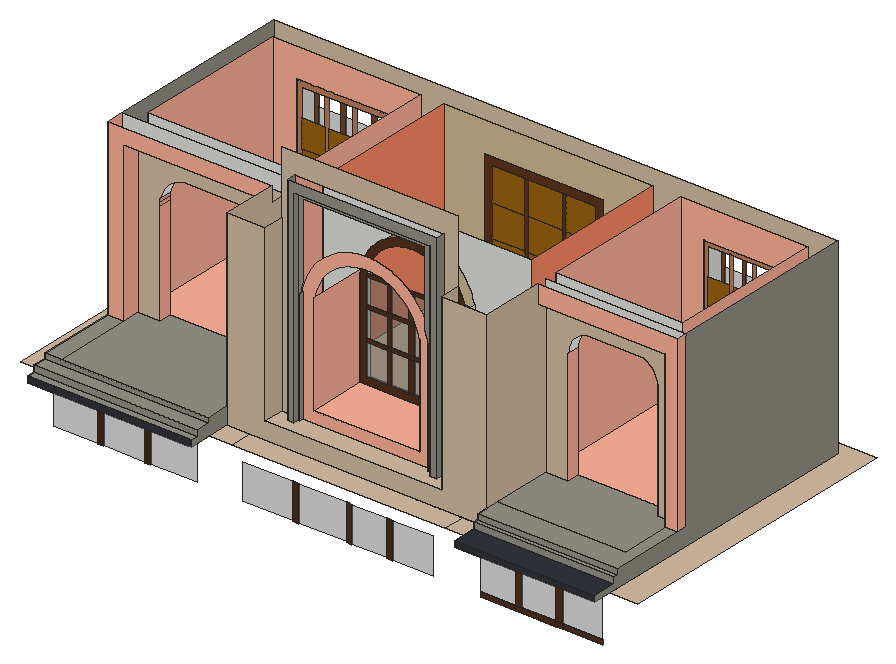
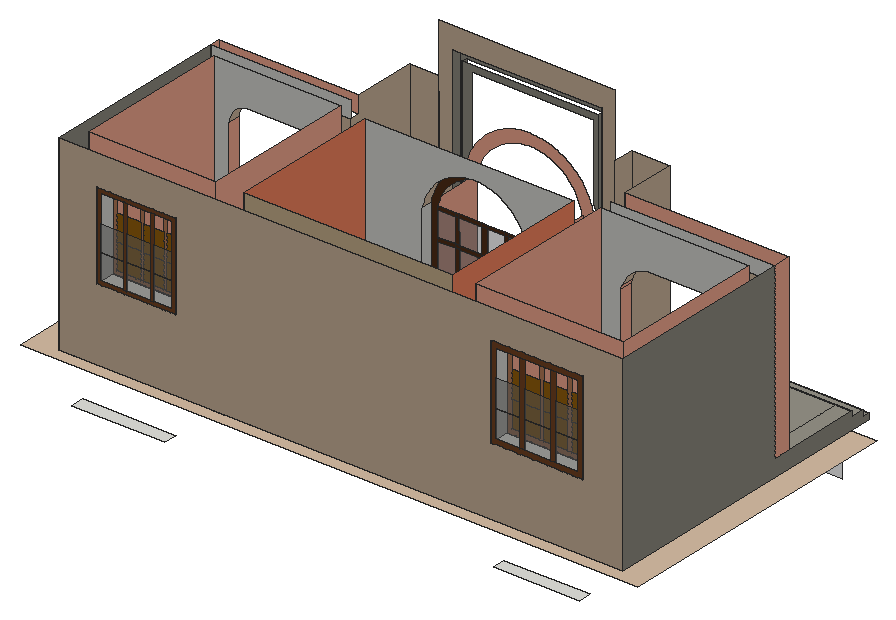
# SketchUp Ruby script. Lengths in inches.
U = 1.inch
M = Sketchup.active_model
def pt(a) = Geom::Point3d.new(a.map { |v| v * U })
def face(e, loops, mat)
  f = e.add_face(loops[0].map { |a| pt(a) })
  loops[1..].each { |l| e.add_face(l.map { |a| pt(a) }).erase! }
  f.material = f.back_material = mat if mat
  f
end
# faces: each face lists its corners as indices into pts; further lists are holes
def faces(e, pts, list, mat = nil) = list.each { |f| face(e, (f[0].is_a?(Array) ? f : [f]).map { |l| l.map { |i| pts[i] } }, mat) }
# xy, xz, yz: faces in a plane at the given z, y or x. An outline is a flat list of corners, or four numbers for a rectangle; further outlines are holes
def ring(l) = l.size == 4 ? [[l[0], l[1]], [l[2], l[1]], [l[2], l[3]], [l[0], l[3]]] : l.each_slice(2).to_a
def flat(e, list, mat, &to3) = list.each { |f| face(e, (f[0].is_a?(Array) ? f : [f]).map { |l| ring(l).map { |u, v| to3.(u, v) } }, mat) }
def xy(e, z, list, mat = nil) = flat(e, list, mat) { |x, y| [x, y, z] }
def xz(e, y, list, mat = nil) = flat(e, list, mat) { |x, z| [x, y, z] }
def yz(e, x, list, mat = nil) = flat(e, list, mat) { |y, z| [x, y, z] }
def lines(e, pts, list) = list.each { |a, b| e.add_line(pt(pts[a]), pt(pts[b])) }
# prism: a flat outline (further loops are holes) pulled along v
def prism(e, loops, v, mat = nil)
  f = face(e, loops, mat); d = Geom::Vector3d.new(v.map { |x| x * U })
  f.pushpull(f.normal.samedirection?(d) ? d.length : -d.length)
end
def box(e, o, s, mat = nil) = prism(e, [[o, [o[0] + s[0], o[1], o[2]], [o[0] + s[0], o[1] + s[1], o[2]], [o[0], o[1] + s[1], o[2]]]], [0, 0, s[2]], mat)
def at(x, y, z, deg = 0) = Geom::Transformation.translation(pt([x, y, z])) * Geom::Transformation.rotation(ORIGIN, Z_AXIS, deg.degrees)
def axes(o, x, y, z) = Geom::Transformation.new([*x, 0, *y, 0, *z, 0, *pt(o).to_a, 1])
def part(name) = M.definitions.add(name)
# library, detail: a bought-in or finely detailed component or shape, given as its bounding box
def library(name, o, s) = part(name).tap { |d| box(d.entities, o, s) }
def detail(e, o, s) = box(e.add_group.entities, o, s)
def put(e, d, t, mat = nil) = e.add_instance(d, t).tap { |i| i.material = mat if mat }
def group(e, t, mat = nil) = e.add_group.tap { |g| g.transformation = t; g.material = mat if mat }.entities
root = M.entities
M.materials.add("[Blinds Wood Light]").color = [155, 100, 14]
M.materials.add("[Color B02]").color = [255, 178, 153]
M.materials.add("[Color B03]").color = [255, 140, 101]
M.materials.add("[Formica Beige]").color = [211, 187, 149]
M.materials.add("[Formica Graystone]").color = [149, 146, 135]
M.materials.add("[Formica Laminate Dark]").color = [50, 53, 60]
M.materials.add("[Formica Laminate Light]").color = [213, 189, 164]
M.materials.add("[Translucent Glass Gray]").color = [128, 128, 128]
M.materials["[Translucent Glass Gray]"].alpha = 0.5
M.materials.add("[Wood Cherry Original]").color = [152, 86, 42]
M.materials.add("[Wood Veneer 01]").color = [71, 41, 22]
M.materials.add("[Wood Veneer 01]1").color = [84, 49, 25]
M.materials.add("[Wood Veneer 01]2").color = [94, 55, 29]
M.materials.add("[Wood Veneer 01]3").color = [84, 49, 25]
M.materials.add("[Wood Veneer 01]4").color = [79, 46, 24]
M.materials.add("[Wood Veneer 01]5").color = [120, 70, 37]
M.materials.add("[Wood Veneer 02]").color = [190, 128, 91]
xy(root,103.85,[[328.4,583.14,393.03,592.14]])
xy(root,106.46,[[40.61,583.14,100.11,592.14]])
xy(root,129,[[128.66,369.56,131.42,385.12],[128.66,385.12,128.66,583.14,146.72,583.14,146.72,400.56,131.42,400.56,131.42,385.12],[311.91,385.12,311.91,400.56,294.66,400.56,294.66,583.14,314.84,583.14,314.84,385.12],[146.72,474.18,294.66,484.13],[146.72,474.18,294.66,484.13]])
xy(root,129,[[17.625,385.12,128.66,583.14],[314.84,385.12,409.38,583.14]],"[Color B02]")
xy(root,129,[[17.625,369.56,128.66,385.12],[311.91,372.18,314.84,385.12],[314.84,372.18,409.38,385.12]],"[Formica Laminate Dark]")
xy(root,129,[[0,385.12,17.625,385.12,17.625,583.14,409.38,583.14,409.38,385.12,428.94,385.12,428.94,592.14,0,592.14],[131.42,385.12,146.72,400.56],[146.72,385.12,294.66,400.56],[294.66,385.12,311.91,400.56]],"[Formica Laminate Light]")
xy(root,129,[[146.72,400.56,294.66,474.18],[146.72,484.13,294.66,583.14]],"[Wood Cherry Original]")
xy(root,133.17,[[311.91,372.18,409.38,388.75]],"[Formica Laminate Dark]")
xy(root,133.35,[[17.625,369.56,131.42,374.93]],"[Formica Graystone]")
xy(root,137.33,[[311.91,388.75,409.38,392.06]],"[Formica Graystone]")
xy(root,137.7,[[17.625,374.93,131.42,384.31]],"[Formica Graystone]")
xy(root,141,[[17.625,438.8,28.78,451.42],[400.54,444.11,409.38,451.42]])
xy(root,141,[[28.78,459.89,131.42,568.57],[311.91,459.89,400.54,568.57]],"[Color B02]")
xy(root,141,[[147.71,463.02,292.81,568.57]],"[Formica Beige]")
xy(root,141,[[17.625,384.31,28.78,438.8],[28.78,384.31,131.42,384.31,131.42,451.42,117.53,451.42,117.53,459.89,43.6875,459.89,43.6875,451.42,28.78,451.42],[311.91,392.06,409.38,392.06,409.38,444.11,400.54,444.11,400.54,409.77,311.91,409.77],[311.91,409.77,400.54,409.77,400.54,451.42,389.71,451.42,389.71,459.89,327.58,459.89,327.58,451.42,311.91,451.42]],"[Formica Graystone]")
xy(root,141,[[157.59,400.56,280.13,400.56,280.13,414.84,270.12,414.84,270.12,408.78,265.76,408.78,265.76,412.53,261.39,412.53,261.39,414.84,172.21,414.84,172.21,412.53,170.76,412.53,170.76,408.78,166.89,408.78,166.89,414.84,157.59,414.84]],"[Formica Laminate Light]")
xy(root,149.01,[[180.21,454.92,253.39,463.02]])
xy(root,149.01,[[180.21,414.84,253.39,454.92]],"[Color B02]")
xy(root,176.09,[[45.27,568.57,109.65,583.14]])
xy(root,178.98,[[327.9375,568.57,383.25,583.14]])
xz(root,369.56,[[17.625,129,131.42,133.35]],"[Formica Laminate Dark]")
xz(root,372.18,[[311.91,129,409.38,133.17]],"[Formica Laminate Dark]")
xz(root,374.93,[[17.625,133.35,131.42,137.7]],"[Formica Graystone]")
xz(root,384.31,[[17.625,137.7,131.42,141]],"[Formica Graystone]")
xz(root,385.12,[[154.41,96.38,189.27,121.31],[193.22,96.38,226.58,121.31],[230.53,96.38,254.8,121.31],[258.75,96.38,286.96,121.31],[22.98,96.89,53.7,123.64],
  [57.87,96.89,86.41,123.64],[90.59,96.89,123.3,123.64],[319.73,98.41,344.24,124.11],[348.55,98.41,372.21,124.11],[376.51,98.41,404.48,124.11]],"[Translucent Glass Gray]")
xz(root,385.12,[[53.7,96.89,57.87,123.64],[86.41,96.89,90.59,123.64]],"[Wood Veneer 01]")
xz(root,385.12,[[319.73,95.2,344.24,98.41],[344.24,95.2,348.55,98.41],[348.55,95.2,372.21,98.41],[372.21,95.2,376.51,98.41],[376.51,95.2,404.48,98.41],
  [344.24,98.41,348.55,124.11],[372.21,98.41,376.51,124.11]],"[Wood Veneer 01]1")
xz(root,385.12,[[189.27,96.38,193.22,121.31],[226.58,96.38,230.53,121.31],[254.8,96.38,258.75,121.31]],"[Wood Veneer 01]4")
xz(root,388.75,[[311.91,133.17,409.38,137.33]],"[Formica Graystone]")
xz(root,392.06,[[311.91,137.33,409.38,141]],"[Formica Graystone]")
xz(root,400.56,[[131.42,129,311.91,129,311.91,261,280.13,261,280.13,141,157.59,141,157.59,261,131.42,261]],"[Formica Laminate Light]")
xz(root,408.78,[[166.89,141,170.76,141,170.76,284,265.76,284,265.76,141,270.12,141,270.12,290.79,166.89,290.79]],"[Formica Graystone]")
xz(root,412.53,[[170.76,141,172.21,141,172.21,219.8125,172.61,221.89,173.11,223.94,173.71,225.97,174.14,227.22,174.14,279.69,259.2,279.69,259.2,227.97,259.89,225.97,260.49,223.94,260.99,221.89,261.39,219.8125,261.39,141,265.76,141,265.76,284,170.76,284]],"[Formica Graystone]")
xz(root,414.84,[[[172.21,141,261.39,141,261.39,219.8125,260.99,221.89,260.49,223.94,259.89,225.97,259.2,227.97,258.42,229.93,257.55,231.85,256.58,233.73,255.53,235.57,254.4,237.35,253.18,239.08,251.89,240.75,250.52,242.36,249.07,243.9,247.56,245.375,245.97,246.77,244.33,248.1,242.62,249.34,240.86,250.51,239.04,251.59,237.18,252.59,235.27,253.49,233.32,254.3125,231.33,255.04,229.32,255.67,227.27,256.21,225.21,256.65,223.12,256.99,221.02,257.24,218.91,257.39,216.8,257.44,214.6875,257.39,212.58,257.24,210.48,256.99,208.39,256.65,206.33,256.21,204.28,255.67,202.27,255.04,200.28,254.3125,198.33,253.49,196.42,252.59,194.56,251.59,192.74,250.51,190.98,249.34,189.27,248.1,187.63,246.77,186.04,245.375,184.53,243.9,183.08,242.36,181.71,240.75,180.42,239.08,179.2,237.35,178.07,235.57,177.02,233.73,176.05,231.85,175.18,229.93,174.4,227.97,174.14,227.22,173.71,225.97,173.11,223.94,172.61,221.89,172.21,219.8125],[180.21,149.01,180.21,219.04,180.43,220.17,180.84,221.86,181.34,223.53,181.9,225.17,182.55,226.79,183.27,228.375,184.06,229.92,184.92,231.43,185.86,232.9,186.86,234.32,187.92,235.7,189.05,237.02,190.24,238.29,191.49,239.5,192.79,240.65,194.15,241.74,195.55,242.77,197,243.73,198.5,244.62,200.03,245.4375,201.6,246.18,203.21,246.86,204.84,247.45,206.5,247.97,208.18,248.42,209.88,248.78,211.6,249.0625,213.33,249.27,215.0625,249.39,216.8,249.43,218.54,249.39,220.27,249.27,222,249.0625,223.72,248.78,225.42,248.42,227.1,247.97,228.76,247.45,230.39,246.86,232,246.18,233.57,245.4375,235.1,244.62,236.6,243.73,238.05,242.77,239.45,241.74,240.81,240.65,242.11,239.5,243.36,238.29,244.55,237.02,245.68,235.7,246.74,234.32,247.74,232.9,248.68,231.43,249.54,229.92,250.33,228.375,251.05,226.79,251.7,225.17,252.26,223.53,252.76,221.86,253.17,220.17,253.39,219.04,253.39,149.01]]],"[Color B02]")
xz(root,414.84,[[157.59,141,166.89,141,166.89,290.79,270.12,290.79,270.12,141,280.13,141,280.13,305.4375,157.59,305.4375]],"[Formica Laminate Light]")
xz(root,438.8,[[17.625,141,28.78,141,28.78,250.57,131.42,250.57,131.42,261,17.625,261]],"[Color B02]")
xz(root,444.11,[[400.54,141,409.38,141,409.38,261,311.91,261,311.91,249.06,400.54,249.06]],"[Color B02]")
xz(root,451.42,[[17.625,141,17.625,261,131.42,261,131.42,250.57,28.78,250.57,28.78,141],[400.54,141,400.54,249.06,311.91,249.06,311.91,261,409.38,261,409.38,141]])
xz(root,451.42,[[28.78,141,43.6875,141,43.6875,212.49,43.82,214.8,44.2,217.08,44.84,219.3,45.72,221.44,46.83,223.47,48.16,225.36,49.6875,227.1,51.4,228.65,53.28,230,55.3,231.14,57.43,232.04,59.64,232.71,100.125,232.71,102.18,232.08,104.18,231.28,106.1,230.3,107.92,229.15,109.63,227.85,111.22,226.4,112.67,224.81,113.98,223.1,115.12,221.27,116.1,219.36,116.91,217.36,117.53,215.3,117.53,141,131.42,141,131.42,250.57,28.78,250.57],[311.91,141,327.58,141,327.58,219.87,327.69,221.79,328.03,223.69,328.58,225.53,329.35,227.29,330.3125,228.96,331.47,230.5,332.79,231.9,334.27,233.13,335.88,234.18,337.6,235.04,339.41,235.6875,341.29,236.125,376.4,236.125,378.14,236.01,379.85,235.67,381.49,235.11,383.05,234.34,384.5,233.375,385.81,232.23,386.96,230.92,387.92,229.47,388.69,227.91,389.25,226.26,389.59,224.56,389.71,222.82,389.71,141,400.54,141,400.54,249.06,311.91,249.06]],"[Formica Laminate Light]")
xz(root,454.92,[[248.46,153.83,248.57,175.58],[248.46,175.58,248.57,178.15],[248.46,178.15,248.57,196.59],[248.46,196.59,248.57,199.01],[248.46,199.01,248.57,216.28],
  [248.46,216.28,248.57,218.57]])
xz(root,454.92,[[185.03,153.83,199.57,175.58],[202.13,153.83,213.78,153.83,213.78,175.58,202.15,175.58],[218.3125,153.83,233.38,153.83,233.55,175.58,218.3125,175.58],[236.52,153.83,248.46,175.58],[185.03,178.15,199.57,196.59],
  [202.15,178.15,213.78,178.15,213.78,196.59,202.17,196.59],[218.3125,178.15,233.57,178.15,233.71,196.59,218.3125,196.59],[236.52,178.15,248.46,196.59],[185.03,199.01,199.57,216.28],[202.17,199.01,213.78,199.01,213.78,216.28,202.18,216.28],
  [218.3125,199.01,233.73,199.01,233.86,216.28,218.3125,216.28],[236.52,199.01,248.46,216.28]],"[Translucent Glass Gray]")
xz(root,454.92,[[[180.21,149.01,253.39,149.01,253.39,219.04,253.17,220.17,252.76,221.86,252.26,223.53,251.7,225.17,251.05,226.79,250.33,228.375,249.54,229.92,248.68,231.43,247.74,232.9,246.74,234.32,245.68,235.7,244.55,237.02,243.36,238.29,242.11,239.5,240.81,240.65,239.45,241.74,238.05,242.77,236.6,243.73,235.1,244.62,233.57,245.4375,232,246.18,230.39,246.86,228.76,247.45,227.1,247.97,225.42,248.42,223.72,248.78,222,249.0625,220.27,249.27,218.54,249.39,216.8,249.43,215.0625,249.39,213.33,249.27,211.6,249.0625,209.88,248.78,208.18,248.42,206.5,247.97,204.84,247.45,203.21,246.86,201.6,246.18,200.03,245.4375,198.5,244.62,197,243.73,195.55,242.77,194.15,241.74,192.79,240.65,191.49,239.5,190.24,238.29,189.05,237.02,187.92,235.7,186.86,234.32,185.86,232.9,184.92,231.43,184.06,229.92,183.27,228.375,182.55,226.79,181.9,225.17,181.34,223.53,180.84,221.86,180.43,220.17,180.21,219.04],[185.03,153.83,185.03,219.14,185.14,219.14,185.5,220.61,185.93,222.0625,186.42,223.49,186.99,224.9,187.61,226.28,188.3,227.625,189.05,228.9375,189.86,230.22,190.74,231.46,191.66,232.65,192.65,233.8,193.68,234.91,194.77,235.96,195.9,236.97,197.08,237.91,198.3,238.81,199.57,239.64,200.87,240.42,202.2,241.13,203.57,241.78,204.97,242.37,206.39,242.89,207.83,243.34,209.3,243.72,210.78,244.04,212.27,244.29,213.78,244.46,215.29,244.57,216.8,244.6,218.3125,244.57,219.82,244.46,221.33,244.29,222.82,244.04,224.3,243.72,225.77,243.34,227.21,242.89,228.63,242.37,230.03,241.78,231.4,241.13,232.73,240.42,234.03,239.64,235.3,238.81,236.52,237.91,237.7,236.97,238.83,235.96,239.92,234.91,240.95,233.8,241.9375,232.65,242.86,231.46,243.73,230.22,244.55,228.9375,245.3,227.625,245.99,226.28,246.61,224.9,247.17,223.49,247.67,222.0625,248.1,220.61,248.46,219.14,248.57,218.57,248.57,153.83]],[199.57,153.83,202.13,153.83,202.15,175.58,199.57,175.58],[213.78,153.83,218.3125,175.58],[233.38,153.83,236.52,153.83,236.52,175.58,233.55,175.58],[185.03,175.58,199.57,178.15],
  [199.57,175.58,202.15,178.15],[202.15,175.58,213.78,178.15],[213.78,175.58,218.3125,178.15],[218.3125,175.58,233.55,175.58,233.57,178.15,218.3125,178.15],[233.55,175.58,236.52,175.58,236.52,178.15,233.57,178.15],
  [236.52,175.58,248.46,178.15],[199.57,178.15,202.15,178.15,202.17,196.59,199.57,196.59],[213.78,178.15,218.3125,196.59],[233.57,178.15,236.52,178.15,236.52,196.59,233.71,196.59],[185.03,196.59,199.57,199.01],
  [199.57,196.59,202.17,199.01],[202.17,196.59,213.78,199.01],[213.78,196.59,218.3125,199.01],[218.3125,196.59,233.71,196.59,233.73,199.01,218.3125,199.01],[233.71,196.59,236.52,196.59,236.52,199.01,233.73,199.01],
  [236.52,196.59,248.46,199.01],[199.57,199.01,202.17,199.01,202.18,216.28,199.57,216.28],[213.78,199.01,218.3125,216.28],[233.73,199.01,236.52,199.01,236.52,216.28,233.86,216.28],[185.03,216.28,199.57,218.57],
  [199.57,216.28,202.18,218.57],[202.18,216.28,213.78,218.57],[213.78,216.28,218.3125,218.57],[218.3125,216.28,233.86,216.28,233.875,218.57,218.3125,218.57],[233.86,216.28,236.52,216.28,236.52,218.57,233.875,218.57],
  [236.52,216.28,248.46,218.57]],"[Wood Veneer 01]3")
xz(root,459.89,[[28.78,141,28.78,261,131.42,261,131.42,141,117.53,141,117.53,215.3,116.91,217.36,116.1,219.36,115.12,221.27,113.98,223.1,112.67,224.81,111.22,226.4,109.63,227.85,107.92,229.15,106.1,230.3,104.18,231.28,102.18,232.08,100.125,232.71,59.64,232.71,57.43,232.04,55.3,231.14,53.28,230,51.4,228.65,49.6875,227.1,48.16,225.36,46.83,223.47,45.72,221.44,44.84,219.3,44.2,217.08,43.82,214.8,43.6875,212.49,43.6875,141],[311.91,141,311.91,261,400.54,261,400.54,141,389.71,141,389.71,222.82,389.59,224.56,389.25,226.26,388.69,227.91,387.92,229.47,386.96,230.92,385.81,232.23,384.5,233.375,383.05,234.34,381.49,235.11,379.85,235.67,378.14,236.01,376.4,236.125,341.29,236.125,339.41,235.6875,337.6,235.04,335.88,234.18,334.27,233.13,332.79,231.9,331.47,230.5,330.3125,228.96,329.35,227.29,328.58,225.53,328.03,223.69,327.69,221.79,327.58,219.87,327.58,141]])
xz(root,463.02,[[[147.71,141,292.81,261],[180.21,149.01,253.39,149.01,253.39,219.04,253.17,220.17,252.76,221.86,252.26,223.53,251.7,225.17,251.05,226.79,250.33,228.375,249.54,229.92,248.68,231.43,247.74,232.9,246.74,234.32,245.68,235.7,244.55,237.02,243.36,238.29,242.11,239.5,240.81,240.65,239.45,241.74,238.05,242.77,236.6,243.73,235.1,244.62,233.57,245.4375,232,246.18,230.39,246.86,228.76,247.45,227.1,247.97,225.42,248.42,223.72,248.78,222,249.0625,220.27,249.27,218.54,249.39,216.8,249.43,215.0625,249.39,213.33,249.27,211.6,249.0625,209.88,248.78,208.18,248.42,206.5,247.97,204.84,247.45,203.21,246.86,201.6,246.18,200.03,245.4375,198.5,244.62,197,243.73,195.55,242.77,194.15,241.74,192.79,240.65,191.49,239.5,190.24,238.29,189.05,237.02,187.92,235.7,186.86,234.32,185.86,232.9,184.92,231.43,184.06,229.92,183.27,228.375,182.55,226.79,181.9,225.17,181.34,223.53,180.84,221.86,180.43,220.17,180.21,219.04]]])
xz(root,568.57,[[181,166.43,203.48,188.79],[206.34,166.43,229.04,188.79],[231.9,166.43,252.66,188.79],[48.75,179.5625,64.6,198.49],[67.24,179.5625,84.0625,198.49],
  [86.71,179.5625,106.17,198.49],[330.49,181.53,345.72,199.64],[348.05,181.53,362.04,199.64],[364.37,181.53,380.69,199.64],[181,188.79,203.48,211.16],
  [206.34,188.79,229.04,211.16],[231.9,188.79,252.66,211.16],[48.75,198.49,64.6,217.42],[67.24,198.49,84.0625,217.42],[86.71,198.49,106.17,217.42],
  [330.49,199.64,345.72,217.74],[348.05,199.64,362.04,217.74],[364.37,199.64,380.69,217.74],[181,211.16,203.48,234.46],[206.34,211.16,229.04,234.46],
  [231.9,211.16,252.66,234.46]],"[Blinds Wood Light]")
xz(root,568.57,[[[28.78,141,131.42,261],[45.27,176.09,109.65,240.46]],[[311.91,141,400.54,261],[327.9375,178.98,383.25,239.54]]],"[Color B02]")
xz(root,568.57,[[[147.71,141,292.81,261],[175.67,161.1,257.99,239.78]]],"[Formica Beige]")
xz(root,568.57,[[[175.67,161.1,257.99,239.78],[181,166.43,252.66,234.46]],[203.48,166.43,206.34,234.46],[229.04,166.43,231.9,234.46]],"[Wood Veneer 01]2")
xz(root,568.57,[[[45.27,176.09,109.65,240.46],[48.75,179.5625,106.17,236.99]],[[327.9375,178.98,383.25,239.54],[330.49,181.53,380.69,236.98]],[64.6,179.5625,67.24,236.99],[84.0625,179.5625,86.71,236.99],[345.72,181.53,348.05,236.98],
  [362.04,181.53,364.37,236.98]],"[Wood Veneer 02]")
xz(root,583.14,[[[17.625,129,409.38,261],[45.27,176.09,109.65,240.46],[327.9375,178.98,383.25,239.54]]],"[Formica Laminate Light]")
xz(root,583.14,[[49,179.82,64.12,199.01],[67.33,179.82,85.93,199.01],[89.14,179.82,105.92,199.01],[330.83,181.87,343.23,199.66],[345.56,181.87,362.04,199.66],
  [364.37,181.87,380.36,199.66],[49,199.01,64.12,218.21],[67.33,199.01,85.93,218.21],[89.14,199.01,105.92,218.21],[330.83,199.66,343.23,217.46],
  [345.56,199.66,362.04,217.46],[364.37,199.66,380.36,217.46]],"[Translucent Glass Gray]")
xz(root,583.14,[[[45.27,176.09,109.65,240.46],[49,179.82,105.92,236.74]],[[327.9375,178.98,383.25,239.54],[330.83,181.87,380.36,236.65]],[64.12,179.82,67.33,236.74],[85.93,179.82,89.14,236.74],[343.23,181.87,345.56,236.65],
  [362.04,181.87,364.37,236.65]],"[Wood Veneer 01]5")
yz(root,17.625,[[438.8,141,451.42,261]],"[Color B02]")
yz(root,17.625,[[369.56,129,369.56,133.35,374.93,133.35,374.93,137.7,384.31,137.7,384.31,141,451.42,141,451.42,261,583.14,261,583.14,129]],"[Formica Graystone]")
yz(root,28.78,[[438.8,141,451.42,250.57],[459.89,141,568.57,261]],"[Color B02]")
yz(root,43.6875,[[451.42,141,459.89,212.49]],"[Color B02]")
yz(root,45.27,[[568.57,176.09,583.14,240.46]])
yz(root,109.65,[[568.57,176.09,583.14,240.46]])
yz(root,117.53,[[451.42,141,459.89,215.3]],"[Color B02]")
yz(root,131.42,[[459.89,141,568.57,261]],"[Color B02]")
yz(root,131.42,[[369.56,129,400.56,129,400.56,141,384.31,141,384.31,137.7,374.93,137.7,374.93,133.35,369.56,133.35]],"[Formica Graystone]")
yz(root,131.42,[[400.56,141,400.56,261,438.8,261,438.8,250.57,451.42,250.57,451.42,141]],"[Formica Laminate Light]")
yz(root,147.71,[[463.02,141,568.57,261]],"[Color B03]")
yz(root,157.59,[[400.56,141,414.84,261]],"[Formica Laminate Light]")
yz(root,166.89,[[408.78,141,414.84,290.79]],"[Formica Graystone]")
yz(root,170.76,[[408.78,141,412.53,284]],"[Formica Graystone]")
yz(root,172.21,[[412.53,141,414.84,219.8125]],"[Formica Graystone]")
yz(root,180.21,[[454.92,149.01,463.02,219.04]])
yz(root,180.21,[[414.84,149.01,454.92,219.04]],"[Color B02]")
yz(root,253.39,[[454.92,149.01,463.02,219.04]])
yz(root,253.39,[[414.84,149.01,454.92,219.04]],"[Color B02]")
yz(root,261.39,[[412.53,141,414.84,219.8125]],"[Formica Graystone]")
yz(root,265.76,[[408.78,141,412.53,284]],"[Formica Graystone]")
yz(root,270.12,[[408.78,141,414.84,290.79]],"[Formica Graystone]")
yz(root,280.13,[[400.56,141,414.84,261]],"[Formica Laminate Light]")
yz(root,292.81,[[463.02,141,568.57,261]],"[Color B03]")
yz(root,311.91,[[459.89,141,568.57,261]],"[Color B02]")
yz(root,311.91,[[372.18,129,400.56,133.17]],"[Formica Laminate Dark]")
yz(root,311.91,[[388.75,133.17,400.56,137.33],[392.06,137.33,400.56,141],[400.56,141,451.42,141,451.42,249.06,444.11,249.06,444.11,261,400.56,261]],"[Formica Laminate Light]")
yz(root,327.58,[[451.42,141,459.89,219.87]],"[Color B02]")
yz(root,327.9375,[[568.57,178.98,583.14,239.54]])
yz(root,383.25,[[568.57,178.98,583.14,239.54]])
yz(root,389.71,[[451.42,141,459.89,222.82]],"[Color B02]")
yz(root,400.54,[[444.11,141,451.42,249.06],[459.89,141,568.57,261]],"[Color B02]")
yz(root,409.38,[[444.11,141,451.42,261]],"[Color B02]")
yz(root,409.38,[[372.18,129,583.14,129,583.14,261,451.42,261,451.42,141,392.06,141,392.06,137.33,388.75,137.33,388.75,133.17,372.18,133.17]],"[Formica Graystone]")
p = [[200.25,474.18,95.625],[198.94,474.18,94.47],[198.94,484.13,94.47],[200.25,484.13,95.625],[240.1,474.18,94.47],[238.79,474.18,95.625],
  [238.79,484.13,95.625],[240.1,484.13,94.47],[201.62,474.18,96.7],[201.62,484.13,96.7],[237.42,474.18,96.7],[237.42,484.13,96.7],
  [203.05,474.18,97.69],[203.05,484.13,97.69],[235.99,474.18,97.69],[235.99,484.13,97.69],[204.54,474.18,98.6],[204.54,484.13,98.6],
  [234.5,474.18,98.6],[234.5,484.13,98.6],[206.07,474.18,99.42],[206.07,484.13,99.42],[232.96,474.18,99.42],[232.96,484.13,99.42],
  [207.66,474.18,100.15],[207.66,484.13,100.15],[231.38,474.18,100.15],[231.38,484.13,100.15],[209.28,474.18,100.79],[209.28,484.13,100.79],
  [229.76,474.18,100.79],[229.76,484.13,100.79],[210.93,474.18,101.33],[210.93,484.13,101.33],[228.11,474.18,101.33],[228.11,484.13,101.33],
  [212.61,474.18,101.78],[212.61,484.13,101.78],[226.42,474.18,101.78],[226.42,484.13,101.78],[214.32,474.18,102.13],[214.32,484.13,102.13],
  [224.72,474.18,102.13],[224.72,484.13,102.13],[216.04,474.18,102.38],[216.04,484.13,102.38],[223,474.18,102.38],[223,484.13,102.38],
  [217.78,474.18,102.53],[217.78,484.13,102.53],[221.26,474.18,102.53],[221.26,484.13,102.53],[219.52,474.18,102.58],[219.52,484.13,102.58],
  [43.82,451.42,214.8],[43.6875,451.42,212.49],[43.6875,459.89,212.49],[43.82,459.89,214.8],[44.2,451.42,217.08],[44.2,459.89,217.08],
  [117.53,451.42,215.3],[116.91,451.42,217.36],[116.91,459.89,217.36],[117.53,459.89,215.3]]
faces(root,p,[[0,1,2,3],[4,5,6,7],[8,0,3,9],[5,10,11,6],[12,8,9,13],[10,14,15,11],[16,12,13,17],[14,18,19,15],
  [20,16,17,21],[18,22,23,19],[24,20,21,25],[22,26,27,23],[28,24,25,29],[26,30,31,27],[32,28,29,33],[30,34,35,31],
  [36,32,33,37],[34,38,39,35],[40,36,37,41],[38,42,43,39],[44,40,41,45],[42,46,47,43],[48,44,45,49],[46,50,51,47],
  [52,48,49,53],[50,52,53,51]],"[Formica Laminate Dark]")
faces(root,p,[[54,55,56,57],[58,54,57,59],[60,61,62,63]],"[Color B02]")
